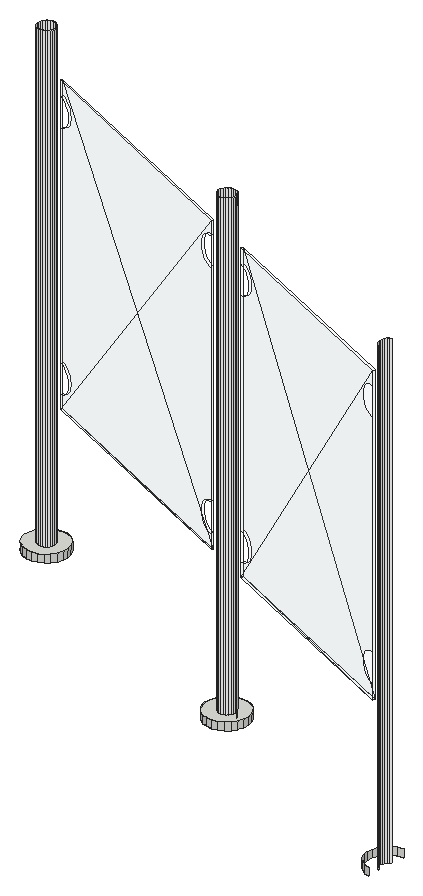
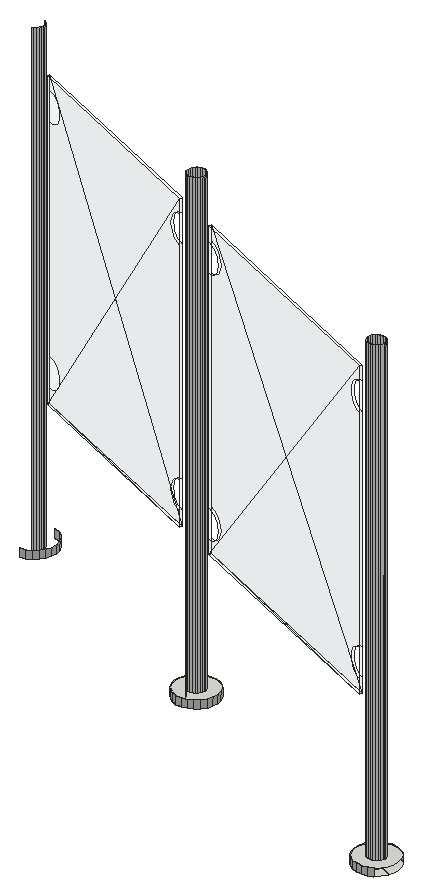
# SketchUp Ruby script. Lengths in inches.
U = 1.inch
M = Sketchup.active_model
def pt(a) = Geom::Point3d.new(a.map { |v| v * U })
def face(e, loops, mat)
  f = e.add_face(loops[0].map { |a| pt(a) })
  loops[1..].each { |l| e.add_face(l.map { |a| pt(a) }).erase! }
  f.material = f.back_material = mat if mat
  f
end
# faces: each face lists its corners as indices into pts; further lists are holes
def faces(e, pts, list, mat = nil) = list.each { |f| face(e, (f[0].is_a?(Array) ? f : [f]).map { |l| l.map { |i| pts[i] } }, mat) }
# xy, xz, yz: faces in a plane at the given z, y or x. An outline is a flat list of corners, or four numbers for a rectangle; further outlines are holes
def ring(l) = l.size == 4 ? [[l[0], l[1]], [l[2], l[1]], [l[2], l[3]], [l[0], l[3]]] : l.each_slice(2).to_a
def flat(e, list, mat, &to3) = list.each { |f| face(e, (f[0].is_a?(Array) ? f : [f]).map { |l| ring(l).map { |u, v| to3.(u, v) } }, mat) }
def xy(e, z, list, mat = nil) = flat(e, list, mat) { |x, y| [x, y, z] }
def xz(e, y, list, mat = nil) = flat(e, list, mat) { |x, z| [x, y, z] }
def yz(e, x, list, mat = nil) = flat(e, list, mat) { |y, z| [x, y, z] }
def lines(e, pts, list) = list.each { |a, b| e.add_line(pt(pts[a]), pt(pts[b])) }
# prism: a flat outline (further loops are holes) pulled along v
def prism(e, loops, v, mat = nil)
  f = face(e, loops, mat); d = Geom::Vector3d.new(v.map { |x| x * U })
  f.pushpull(f.normal.samedirection?(d) ? d.length : -d.length)
end
def box(e, o, s, mat = nil) = prism(e, [[o, [o[0] + s[0], o[1], o[2]], [o[0] + s[0], o[1] + s[1], o[2]], [o[0], o[1] + s[1], o[2]]]], [0, 0, s[2]], mat)
def at(x, y, z, deg = 0) = Geom::Transformation.translation(pt([x, y, z])) * Geom::Transformation.rotation(ORIGIN, Z_AXIS, deg.degrees)
def axes(o, x, y, z) = Geom::Transformation.new([*x, 0, *y, 0, *z, 0, *pt(o).to_a, 1])
def part(name) = M.definitions.add(name)
# library, detail: a bought-in or finely detailed component or shape, given as its bounding box
def library(name, o, s) = part(name).tap { |d| box(d.entities, o, s) }
def detail(e, o, s) = box(e.add_group.entities, o, s)
def put(e, d, t, mat = nil) = e.add_instance(d, t).tap { |i| i.material = mat if mat }
def group(e, t, mat = nil) = e.add_group.tap { |g| g.transformation = t; g.material = mat if mat }.entities
root = M.entities
M.materials.add("Glass_Safety_01").color = [204, 235, 244]
M.materials["Glass_Safety_01"].alpha = 0.1
M.materials.add("[Color_000]").color = [255, 255, 255]
xy(root,321.27,[[[808.39,547.68,808.79,547.76,809.16,547.95,809.46,548.22,809.69,548.5625,809.71,548.625,809.82,548.95,809.84,549.36,809.76,549.77,809.58,550.13,809.3,550.44,808.96,550.67,808.57,550.8,808.16,550.82,807.76,550.74,807.39,550.55,807.08,550.28,806.86,549.9375,806.84,549.875,806.73,549.55,806.7,549.14,806.78,548.74,806.97,548.37,807.24,548.06,807.59,547.83,807.98,547.7],[808.32,548.62,808.15,548.63,808,548.68,807.86,548.77,807.75,548.9,807.68,549.04,807.64,549.21,807.65,549.37,807.7,549.5,807.71,549.53,807.8,549.66,807.92,549.77,808.07,549.85,808.23,549.88,808.39,549.87,808.55,549.82,808.69,549.73,808.79,549.6,808.87,549.46,808.9,549.3,808.89,549.13,808.85,549,808.84,548.98,808.75,548.84,808.625,548.73,808.48,548.66]],[809.71,548.625,809.82,548.95,809.84,549.36,809.76,549.77,809.58,550.13,809.3,550.44,808.96,550.67,808.57,550.8,808.16,550.82,807.76,550.74,807.39,550.55,807.08,550.28,806.86,549.9375,806.84,549.875,807.7,549.5,807.71,549.53,807.8,549.66,807.92,549.77,808.07,549.85,808.23,549.88,808.39,549.87,808.55,549.82,808.69,549.73,808.79,549.6,808.87,549.46,808.9,549.3,808.89,549.13,808.85,549],[808.85,549,808.89,549.13,808.9,549.3,808.87,549.46,808.79,549.6,808.69,549.73,808.55,549.82,808.39,549.87,808.23,549.88,808.07,549.85,807.92,549.77,807.8,549.66,807.71,549.53,807.7,549.5],[[787.16,556.92,787.57,557,787.94,557.1875,788.24,557.46,788.47,557.8,788.49,557.87,788.6,558.19,788.625,558.61,788.54,559.01,788.36,559.375,788.08,559.68,787.74,559.91,787.35,560.04,786.94,560.0625,786.54,559.98,786.17,559.8,785.86,559.52,785.64,559.18,785.51,558.79,785.48,558.38,785.5625,557.98,785.75,557.61,786.02,557.3,786.36,557.08,786.75,556.95],[787.1,557.86,786.93,557.875,786.78,557.93,786.64,558.02,786.53,558.14,786.46,558.29,786.42,558.45,786.43,558.61,786.48,558.74,786.49,558.77,786.58,558.9,786.7,559.01,786.85,559.09,787.01,559.12,787.17,559.11,787.33,559.06,787.46,558.97,787.57,558.85,787.65,558.7,787.68,558.54,787.67,558.375,787.63,558.24,787.62,558.22,787.53,558.08,787.41,557.97,787.26,557.9]],[788.49,557.87,788.6,558.19,788.625,558.61,788.54,559.01,788.36,559.375,788.08,559.68,787.74,559.91,787.35,560.04,786.94,560.0625,786.54,559.98,786.17,559.8,785.86,559.52,785.64,559.18,785.62,559.12,786.48,558.74,786.49,558.77,786.58,558.9,786.7,559.01,786.85,559.09,787.01,559.12,787.17,559.11,787.33,559.06,787.46,558.97,787.57,558.85,787.65,558.7,787.68,558.54,787.67,558.375,787.63,558.24],
  [787.63,558.24,787.67,558.375,787.68,558.54,787.65,558.7,787.57,558.85,787.46,558.97,787.33,559.06,787.17,559.11,787.01,559.12,786.85,559.09,786.7,559.01,786.58,558.9,786.49,558.77,786.48,558.74]])
xy(root,321.27,[[808.32,548.62,808.48,548.66,808.625,548.73,808.75,548.84,808.84,548.98,808.85,549,807.7,549.5,807.65,549.37,807.64,549.21,807.68,549.04,807.75,548.9,807.86,548.77,808,548.68,808.15,548.63],[787.1,557.86,787.26,557.9,787.41,557.97,787.53,558.08,787.62,558.22,787.63,558.24,786.48,558.74,786.43,558.61,786.42,558.45,786.46,558.29,786.53,558.14,786.64,558.02,786.78,557.93,786.93,557.875]],"[Color_000]")
xy(root,321.86,[[808.39,547.68,808.79,547.76,809.16,547.95,809.46,548.22,809.69,548.5625,809.82,548.95,809.84,549.36,809.76,549.77,809.58,550.13,809.3,550.44,808.96,550.67,808.57,550.8,808.16,550.82,807.76,550.74,807.39,550.55,807.08,550.28,806.86,549.9375,806.73,549.55,806.7,549.14,806.78,548.74,806.97,548.37,807.24,548.06,807.59,547.83,807.98,547.7],[787.16,556.92,787.57,557,787.94,557.1875,788.24,557.46,788.47,557.8,788.6,558.19,788.625,558.61,788.54,559.01,788.36,559.375,788.08,559.68,787.74,559.91,787.35,560.04,786.94,560.0625,786.54,559.98,786.17,559.8,785.86,559.52,785.64,559.18,785.51,558.79,785.48,558.38,785.5625,557.98,785.75,557.61,786.02,557.3,786.36,557.08,786.75,556.95]])
xy(root,331.9,[[825.6,541.6,810.04,548.375,810.12,548.55],[825.6,541.6,810.12,548.55,825.67,541.78],[806.58,549.88,788.82,557.62,788.9,557.8],[806.58,549.88,788.9,557.8,806.66,550.06]],"Glass_Safety_01")
p = [[826.58,539.5625,321.27],[826.97,539.43,321.27],[826.97,539.43,321.86],[826.58,539.5625,321.86],[826.24,539.79,321.27],[826.24,539.79,321.86],
  [825.96,540.1,321.27],[825.96,540.1,321.86],[825.78,540.46,321.27],[825.78,540.46,321.86],[826.86,540.5,321.27],[826.99,540.41,321.27],
  [826.99,540.41,357.27],[826.86,540.5,357.27],[825.7,540.87,321.27],[825.7,540.87,321.86],[826.75,540.625,321.27],[826.75,540.625,357.27],
  [826.67,540.77,321.27],[826.67,540.77,357.27],[826.64,540.93,321.27],[826.64,540.93,357.27],[825.72,541.28,321.27],[825.72,541.28,321.86],
  [826.65,541.1,321.27],[826.65,541.1,357.27],[826.7,541.25,321.27],[826.69,541.23,321.27],[826.7,541.25,357.27],[825.85,541.67,321.27],
  [825.83,541.6,321.27],[825.85,541.67,321.86],[826.79,541.39,321.27],[826.79,541.39,357.27],[826.91,541.5,321.27],[826.91,541.5,357.27],
  [827.0625,541.57,321.27],[827.0625,541.57,357.27],[826.08,542.01,321.27],[826.08,542.01,321.86],[826.39,542.28,321.27],[826.39,542.28,321.86],
  [826.75,542.47,321.27],[826.75,542.47,321.86],[827.16,542.55,321.27],[827.16,542.55,321.86],[807.59,547.83,321.27],[807.98,547.7,321.27],
  [807.98,547.7,321.86],[807.59,547.83,321.86],[808.39,547.68,321.27],[808.39,547.68,321.86],[808.79,547.76,321.27],[808.79,547.76,321.86],
  [807.24,548.06,321.27],[807.24,548.06,321.86],[809.16,547.95,321.27],[809.16,547.95,321.86],[809.46,548.22,321.27],[809.46,548.22,321.86],
  [806.97,548.37,321.27],[806.97,548.37,321.86],[809.69,548.5625,321.27],[809.69,548.5625,321.86],[806.78,548.74,321.27],[806.78,548.74,321.86],
  [808,548.68,321.27],[808.15,548.63,321.27],[808.15,548.63,357.27],[808,548.68,357.27],[808.32,548.62,321.27],[808.32,548.62,357.27],
  [808.48,548.66,321.27],[808.48,548.66,357.27],[809.71,548.625,321.27],[809.82,548.95,321.27],[809.82,548.95,321.86],[806.7,549.14,321.27],
  [806.7,549.14,321.86],[807.86,548.77,321.27],[807.86,548.77,357.27],[808.625,548.73,321.27],[808.625,548.73,357.27],[808.75,548.84,321.27],
  [808.75,548.84,357.27],[807.75,548.9,321.27],[807.75,548.9,357.27],[808.84,548.98,321.27],[808.84,548.98,357.27],[807.68,549.04,321.27],
  [807.68,549.04,357.27],[807.64,549.21,321.27],[807.64,549.21,357.27],[808.85,549,321.27],[808.89,549.13,321.27],[808.89,549.13,357.27],
  [809.84,549.36,321.27],[809.84,549.36,321.86],[806.73,549.55,321.27],[806.73,549.55,321.86],[808.9,549.3,321.27],[808.9,549.3,357.27],
  [807.65,549.37,321.27],[807.65,549.37,357.27],[808.87,549.46,321.27],[808.87,549.46,357.27],[807.71,549.53,321.27],[807.7,549.5,321.27],
  [807.71,549.53,357.27],[809.76,549.77,321.27],[809.76,549.77,321.86],[806.86,549.9375,321.27],[806.84,549.875,321.27],[806.86,549.9375,321.86],
  [807.8,549.66,321.27],[807.8,549.66,357.27],[808.79,549.6,321.27],[808.79,549.6,357.27],[808.69,549.73,321.27],[808.69,549.73,357.27],
  [807.92,549.77,321.27],[807.92,549.77,357.27],[808.55,549.82,321.27],[808.55,549.82,357.27],[808.07,549.85,321.27],[808.07,549.85,357.27],
  [808.23,549.88,321.27],[808.23,549.88,357.27],[808.39,549.87,321.27],[808.39,549.87,357.27],[809.58,550.13,321.27],[809.58,550.13,321.86],
  [807.08,550.28,321.27],[807.08,550.28,321.86],[809.3,550.44,321.27],[809.3,550.44,321.86],[807.39,550.55,321.27],[807.39,550.55,321.86],
  [808.96,550.67,321.27],[808.96,550.67,321.86],[807.76,550.74,321.27],[807.76,550.74,321.86],[808.16,550.82,321.27],[808.16,550.82,321.86],
  [808.57,550.8,321.27],[808.57,550.8,321.86],[786.36,557.08,321.27],[786.75,556.95,321.27],[786.75,556.95,321.86],[786.36,557.08,321.86],
  [787.16,556.92,321.27],[787.16,556.92,321.86],[787.57,557,321.27],[787.57,557,321.86],[787.94,557.1875,321.27],[787.94,557.1875,321.86],
  [786.02,557.3,321.27],[786.02,557.3,321.86],[788.24,557.46,321.27],[788.24,557.46,321.86],[788.47,557.8,321.27],[788.47,557.8,321.86],
  [788.49,557.87,321.27],[788.6,558.19,321.27],[788.6,558.19,321.86],[786.64,558.02,321.27],[786.78,557.93,321.27],[786.78,557.93,357.27],
  [786.64,558.02,357.27],[786.93,557.875,321.27],[786.93,557.875,357.27],[787.1,557.86,321.27],[787.1,557.86,357.27],[787.26,557.9,321.27],
  [787.26,557.9,357.27],[787.41,557.97,321.27],[787.41,557.97,357.27],[786.53,558.14,321.27],[786.53,558.14,357.27],[787.53,558.08,321.27],
  [787.53,558.08,357.27],[786.46,558.29,321.27],[786.46,558.29,357.27],[787.62,558.22,321.27],[787.62,558.22,357.27],[787.63,558.24,321.27],
  [787.67,558.375,321.27],[787.67,558.375,357.27],[788.625,558.61,321.27],[788.625,558.61,321.86],[786.42,558.45,321.27],[786.42,558.45,357.27],
  [786.43,558.61,321.27],[786.43,558.61,357.27],[787.68,558.54,321.27],[787.68,558.54,357.27],[787.65,558.7,321.27],[787.65,558.7,357.27],
  [786.49,558.77,321.27],[786.48,558.74,321.27],[786.49,558.77,357.27],[788.54,559.01,321.27],[788.54,559.01,321.86],[787.57,558.85,321.27],
  [787.57,558.85,357.27],[786.58,558.9,321.27],[786.58,558.9,357.27],[787.46,558.97,321.27],[787.46,558.97,357.27],[786.7,559.01,321.27],
  [786.7,559.01,357.27],[786.85,559.09,321.27],[786.85,559.09,357.27],[787.33,559.06,321.27],[787.33,559.06,357.27],[788.36,559.375,321.27],
  [788.36,559.375,321.86],[787.01,559.12,321.27],[787.01,559.12,357.27],[787.17,559.11,321.27],[787.17,559.11,357.27],[788.08,559.68,321.27],
  [788.08,559.68,321.86],[787.74,559.91,321.27],[787.74,559.91,321.86],[786.54,559.98,321.27],[786.17,559.8,321.27],[786.17,559.8,321.86],
  [786.54,559.98,321.86],[787.35,560.04,321.27],[787.35,560.04,321.86],[786.94,560.0625,321.27],[786.94,560.0625,321.86],[810.04,548.375,351.28],
  [810.04,548.375,335.125],[810.29,548.26,335.09],[810.53,548.16,334.98],[810.73,548.07,334.8125],[810.88,548.01,334.59],[810.98,547.96,334.34],
  [811.01,547.95,334.0625],[810.98,547.96,333.79],[810.88,548.01,333.53],[810.73,548.07,333.3125],[810.53,548.16,333.14],[810.29,548.26,333.04],
  [810.04,548.375,333],[810.04,548.375,331.9],[825.6,541.6,354.51],[810.04,548.375,354.51],[810.04,548.375,353.41],[810.29,548.26,353.37],
  [810.53,548.16,353.27],[810.73,548.07,353.1],[810.88,548.01,352.88],[810.98,547.96,352.62],[811.01,547.95,352.35],[810.98,547.96,352.07],
  [810.88,548.01,351.81],[810.73,548.07,351.59],[810.53,548.16,351.43],[810.29,548.26,351.32],[825.6,541.6,331.9],[825.6,541.6,333],
  [825.42,541.67,333],[825.17,541.78,333.04],[824.9375,541.89,333.14],[824.73,541.97,333.3125],[824.58,542.04,333.53],[824.48,542.08,333.79],
  [824.45,542.1,334.0625],[824.48,542.08,334.34],[824.58,542.04,334.59],[824.73,541.97,334.8125],[824.9375,541.89,334.98],[825.17,541.78,335.09],
  [825.42,541.67,335.125],[825.6,541.6,335.125],[825.6,541.6,351.28],[825.42,541.67,351.28],[825.17,541.78,351.32],[824.9375,541.89,351.43],
  [824.73,541.97,351.59],[824.58,542.04,351.81],[824.48,542.08,352.07],[824.45,542.1,352.35],[824.48,542.08,352.62],[824.58,542.04,352.88],
  [824.73,541.97,353.1],[824.9375,541.89,353.27],[825.17,541.78,353.37],[825.42,541.67,353.41],[825.6,541.6,353.41],[825.67,541.78,331.9],
  [825.67,541.78,333],[825.67,541.78,335.125],[825.67,541.78,351.28],[825.67,541.78,353.41],[825.67,541.78,354.51],[810.12,548.55,331.9],
  [810.12,548.55,333],[810.37,548.44,333.04],[810.6,548.34,333.14],[810.81,548.25,333.3125],[810.96,548.1875,333.53],[811.06,548.14,333.79],
  [811.09,548.13,334.0625],[811.06,548.14,334.34],[810.96,548.1875,334.59],[810.81,548.25,334.8125],[810.6,548.34,334.98],[810.37,548.44,335.09],
  [810.12,548.55,335.125],[810.12,548.55,351.28],[810.37,548.44,351.32],[810.6,548.34,351.43],[810.81,548.25,351.59],[810.96,548.1875,351.81],
  [811.06,548.14,352.07],[811.09,548.13,352.35],[811.06,548.14,352.62],[810.96,548.1875,352.88],[810.81,548.25,353.1],[810.6,548.34,353.27],
  [810.37,548.44,353.37],[810.12,548.55,353.41],[810.12,548.55,354.51],[788.82,557.62,351.28],[788.82,557.62,335.125],[789.07,557.51,335.09],
  [789.31,557.4,334.98],[789.51,557.32,334.8125],[789.66,557.25,334.59],[789.76,557.21,334.34],[789.79,557.19,334.0625],[789.76,557.21,333.79],
  [789.66,557.25,333.53],[789.51,557.32,333.3125],[789.31,557.4,333.14],[789.07,557.51,333.04],[788.82,557.62,333],[788.82,557.62,331.9],
  [806.58,549.88,354.51],[788.82,557.62,354.51],[788.82,557.62,353.41],[789.07,557.51,353.37],[789.31,557.4,353.27],[789.51,557.32,353.1],
  [789.66,557.25,352.88],[789.76,557.21,352.62],[789.79,557.19,352.35],[789.76,557.21,352.07],[789.66,557.25,351.81],[789.51,557.32,351.59],
  [789.31,557.4,351.43],[789.07,557.51,351.32],[806.58,549.88,331.9],[806.58,549.88,333],[806.43,549.95,333],[806.18,550.06,333.04],
  [805.94,550.16,333.14],[805.74,550.25,333.3125],[805.58,550.3125,333.53],[805.49,550.36,333.79],[805.45,550.37,334.0625],[805.49,550.36,334.34],
  [805.58,550.3125,334.59],[805.74,550.25,334.8125],[805.94,550.16,334.98],[806.18,550.06,335.09],[806.43,549.95,335.125],[806.58,549.88,335.125],
  [806.58,549.88,351.28],[806.43,549.95,351.28],[806.18,550.06,351.32],[805.94,550.16,351.43],[805.74,550.25,351.59],[805.58,550.3125,351.81],
  [805.49,550.36,352.07],[805.45,550.37,352.35],[805.49,550.36,352.62],[805.58,550.3125,352.88],[805.74,550.25,353.1],[805.94,550.16,353.27],
  [806.18,550.06,353.37],[806.43,549.95,353.41],[806.58,549.88,353.41],[806.66,550.06,331.9],[806.66,550.06,333],[806.66,550.06,335.125],
  [806.66,550.06,351.28],[806.66,550.06,353.41],[806.66,550.06,354.51],[788.9,557.8,331.9],[788.9,557.8,333],[789.15,557.6875,333.04],
  [789.38,557.58,333.14],[789.59,557.5,333.3125],[789.74,557.43,333.53],[789.84,557.39,333.79],[789.87,557.37,334.0625],[789.84,557.39,334.34],
  [789.74,557.43,334.59],[789.59,557.5,334.8125],[789.38,557.58,334.98],[789.15,557.6875,335.09],[788.9,557.8,335.125],[788.9,557.8,351.28],
  [789.15,557.6875,351.32],[789.38,557.58,351.43],[789.59,557.5,351.59],[789.74,557.43,351.81],[789.84,557.39,352.07],[789.87,557.37,352.35],
  [789.84,557.39,352.62],[789.74,557.43,352.88],[789.59,557.5,353.1],[789.38,557.58,353.27],[789.15,557.6875,353.37],[788.9,557.8,353.41],
  [788.9,557.8,354.51],[806.51,550.125,335.125],[806.26,550.24,335.09],[806.02,550.34,334.98],[805.82,550.43,334.8125],[805.66,550.49,334.59],
  [805.57,550.54,334.34],[805.53,550.55,334.0625],[805.57,550.54,333.79],[805.66,550.49,333.53],[805.82,550.43,333.3125],[806.02,550.34,333.14],
  [806.26,550.24,333.04],[806.51,550.125,333],[806.51,550.125,353.41],[806.26,550.24,353.37],[806.02,550.34,353.27],[805.82,550.43,353.1],
  [805.66,550.49,352.88],[805.57,550.54,352.62],[805.53,550.55,352.35],[805.57,550.54,352.07],[805.66,550.49,351.81],[805.82,550.43,351.59],
  [806.02,550.34,351.43],[806.26,550.24,351.32],[806.51,550.125,351.28]]
faces(root,p,[[0,1,2,3],[4,0,3,5],[6,4,5,7],[8,6,7,9],[14,8,9,15],[22,14,15,23],[29,30,22,23,31],[38,29,31,39],
  [40,38,39,41],[42,40,41,43],[44,42,43,45],[46,47,48,49],[47,50,51,48],[50,52,53,51],[54,46,49,55],[52,56,57,53],
  [56,58,59,57],[60,54,55,61],[58,62,63,59],[64,60,61,65],[62,74,75,76,63],[77,64,65,78],[75,96,97,76],[98,77,78,99],
  [96,109,110,97],[111,112,98,99,113],[109,130,131,110],[132,111,113,133],[130,134,135,131],[136,132,133,137],[134,138,139,135],[140,136,137,141],
  [142,140,141,143],[138,144,145,139],[144,142,143,145],[146,147,148,149],[147,150,151,148],[150,152,153,151],[152,154,155,153],[156,146,149,157],
  [154,158,159,155],[158,160,161,159],[160,162,163,164,161],[163,188,189,164],[188,201,202,189],[201,215,216,202],[215,221,222,216],[221,223,224,222],
  [225,226,227,228],[223,229,230,224],[231,225,228,232],[229,231,232,230]])
faces(root,p,[[10,11,12,13],[16,10,13,17],[18,16,17,19],[20,18,19,21],[24,20,21,25],[26,27,24,25,28],[32,26,28,33],[34,32,33,35],
  [36,34,35,37],[66,67,68,69],[67,70,71,68],[70,72,73,71],[79,66,69,80],[72,81,82,73],[81,83,84,82],[85,79,80,86],
  [83,87,88,84],[89,85,86,90],[91,89,90,92],[87,93,94,95,88],[94,100,101,95],[102,91,92,103],[100,104,105,101],[106,107,102,103,108],
  [114,106,108,115],[104,116,117,105],[116,118,119,117],[120,114,115,121],[118,122,123,119],[124,120,121,125],[126,124,125,127],[122,128,129,123],
  [128,126,127,129],[165,166,167,168],[166,169,170,167],[169,171,172,170],[171,173,174,172],[173,175,176,174],[177,165,168,178],[175,179,180,176],
  [181,177,178,182],[179,183,184,180],[183,185,186,187,184],[190,181,182,191],[192,190,191,193],[186,194,195,187],[194,196,197,195],[198,199,192,193,200],
  [196,203,204,197],[205,198,200,206],[203,207,208,204],[209,205,206,210],[211,209,210,212],[207,213,214,208],[217,211,212,218],[219,217,218,220],
  [213,219,220,214]],"[Color_000]")
faces(root,p,[[233,234,235,236,237,238,239,240,241,242,243,244,245,246,247,248,249,250,251,252,253,254,255,256,257,258,259,260,261],[262,263,264,265,266,267,268,269,270,271,272,273,274,275,276,277,278,279,280,281,282,283,284,285,286,287,288,289,290,291,292,248,247],[262,293,294,295,296,297,298,248,292,278,277,263],[299,300,301,302,303,304,305,306,307,308,309,310,311,312,313,314,315,316,317,318,319,320,321,322,323,324,325,326,293],[293,326,298,297,296,295,294],[299,247,246,234,233,250,249,326,325,313,312,300],[327,328,329,330,331,332,333,334,335,336,337,338,339,340,341,342,343,344,345,346,347,348,349,350,351,352,353,354,355],[356,357,358,359,360,361,362,363,364,365,366,367,368,369,370,371,372,373,374,375,376,377,378,379,380,381,382,383,384,385,386,342,341],
  [356,387,388,389,390,391,392,342,386,372,371,357],[393,394,395,396,397,398,399,400,401,402,403,404,405,406,407,408,409,410,411,412,413,414,415,416,417,418,419,420,387],[390,389,421,422,423,424,425,426,427,428,429,430,431,432,433,388,387,420,392,391,434,435,436,437,438,439,440,441,442,443,444,445,446],[393,341,340,328,327,344,343,420,419,407,406,394]],"Glass_Safety_01")
